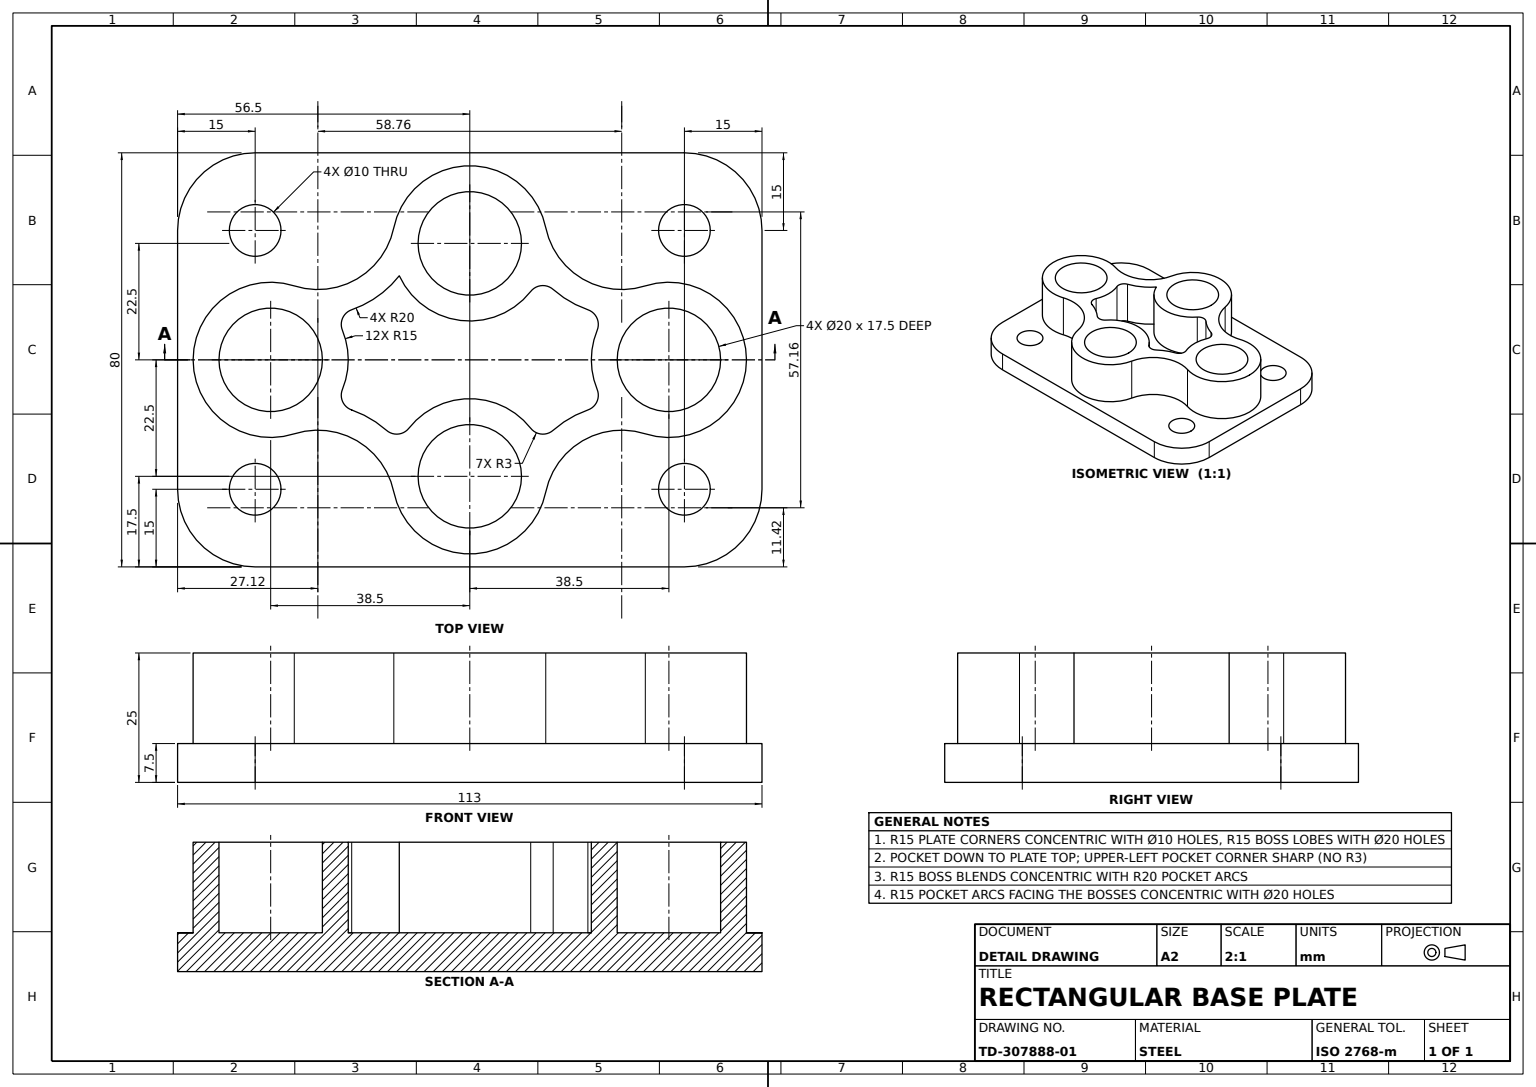
solid
v1 (5.704384,25,-24.627005)
v2 (9.680147,25,-22.833948)
e1 v1 v2 CIRCLE(AX(P(6.845261,25,-21.852406),D(0,-1,0),D(0,0,1)),3)
v3 (5.704384,7.5,-24.627005)
e2 v3 v1 LINE
v4 (9.680147,7.5,-22.833948)
e3 v4 v3 CIRCLE(AX(P(6.845261,7.5,-21.852406),D(0,1,0),D(0,0,1)),3)
e4 v2 v4 LINE
face CYL(AX(P(6.845261,25,-21.852406),D(0,1,0),D(0,0,1)),3) rev [-e1 -e2 -e3 -e4]
v5 (-9.680147,7.5,22.833948)
v6 (-6.845261,7.5,24.852406)
e5 v5 v6 CIRCLE(AX(P(-6.845261,7.5,21.852406),D(0,1,0),D(0,0,1)),3)
v7 (-9.680147,25,22.833948)
e6 v7 v5 LINE
v8 (-6.845261,25,24.852406)
e7 v8 v7 CIRCLE(AX(P(-6.845261,25,21.852406),D(0,-1,0),D(0,0,1)),3)
e8 v6 v8 LINE
face CYL(AX(P(-6.845261,25,21.852406),D(0,1,0),D(0,0,1)),3) rev [-e5 -e6 -e7 -e8]
v9 (0,25,-53.5)
v10 (0,7.5,-53.5)
e9 v9 v10 LINE
v11 (14.289691,25,-33.938781)
e10 v11 v9 CIRCLE(AX(P(0,25,-38.5),D(0,1,0),D(0,0,1)),15)
v12 (14.289691,7.5,-33.938781)
e11 v11 v12 LINE
e12 v12 v10 CIRCLE(AX(P(0,7.5,-38.5),D(0,1,0),D(0,0,1)),15)
face CYL(AX(P(0,25,-38.5),D(0,-1,0),D(0,0,-1)),15) [-e9 -e10 e11 e12]
v13 (25.539691,25,14.688781)
v14 (25.539691,7.5,14.688781)
e13 v13 v14 LINE
v15 (25.539691,7.5,-14.688781)
e14 v14 v15 CIRCLE(AX(P(22.5,7.5,0),D(0,1,0),D(0,0,1)),15)
v16 (25.539691,25,-14.688781)
e15 v16 v15 LINE
e16 v13 v16 CIRCLE(AX(P(22.5,25,0),D(0,1,0),D(0,0,1)),15)
face CYL(AX(P(22.5,25,0),D(0,-1,0),D(0,0,-1)),15) [e13 e14 -e15 -e16]
v17 (0,7.5,28.5)
v18 (0,7.5,48.5)
e17 v17 v18 CIRCLE(AX(P(0,7.5,38.5),D(0,1,0),D(0,0,1)),10)
v19 (0,25,28.5)
e18 v17 v19 LINE
v20 (0,25,48.5)
e19 v19 v20 CIRCLE(AX(P(0,25,38.5),D(0,1,0),D(0,0,1)),10)
e20 v18 v20 LINE
face CYL(AX(P(0,7.5,38.5),D(0,1,0),D(0,0,1)),10) rev [-e17 e18 e19 -e20]
v21 (-40,0,-41.5)
v22 (-25,0,-56.5)
e21 v21 v22 CIRCLE(AX(P(-25,0,-41.5),D(0,-1,0),D(0,0,1)),15)
v23 (-40,7.5,-41.5)
e22 v23 v21 LINE
v24 (-25,7.5,-56.5)
e23 v24 v23 CIRCLE(AX(P(-25,7.5,-41.5),D(0,1,0),D(0,0,1)),15)
e24 v22 v24 LINE
face CYL(AX(P(-25,7.5,-41.5),D(0,-1,0),D(0,0,-1)),15) [-e21 -e22 -e23 -e24]
v25 (25,0,-46.5)
v26 (25,7.5,-46.5)
e25 v25 v26 LINE
v27 (25,7.5,-36.5)
e26 v26 v27 CIRCLE(AX(P(25,7.5,-41.5),D(0,1,0),D(0,0,1)),5)
v28 (25,0,-36.5)
e27 v28 v27 LINE
e28 v25 v28 CIRCLE(AX(P(25,0,-41.5),D(0,1,0),D(0,0,1)),5)
face CYL(AX(P(25,-10,-41.5),D(0,1,0),D(0,0,1)),5) rev [e25 e26 -e27 -e28]
e29 v12 v15 CIRCLE(AX(P(28.579383,7.5,-29.377561),D(0,1,0),D(0,0,1)),15)
e30 v11 v16 CIRCLE(AX(P(28.579383,25,-29.377561),D(0,1,0),D(0,0,1)),15)
face CYL(AX(P(28.579383,25,-29.377561),D(0,-1,0),D(0,0,-1)),15) rev [e15 -e29 -e11 e30]
v29 (14.289691,7.5,33.938781)
e31 v14 v29 CIRCLE(AX(P(28.579383,7.5,29.377561),D(0,1,0),D(0,0,1)),15)
v30 (14.289691,25,33.938781)
e32 v13 v30 CIRCLE(AX(P(28.579383,25,29.377561),D(0,1,0),D(0,0,1)),15)
e33 v30 v29 LINE
face CYL(AX(P(28.579383,25,29.377561),D(0,-1,0),D(0,0,-1)),15) rev [-e31 -e13 e32 e33]
e34 v18 v17 CIRCLE(AX(P(0,7.5,38.5),D(0,1,0),D(0,0,1)),10)
face PLANE(AX(P(0,7.5,38.5),D(0,1,0),D(0,0,1))) [e34 e17]
v31 (-25,0,36.5)
v32 (-25,7.5,36.5)
e35 v31 v32 LINE
v33 (-25,0,46.5)
e36 v33 v31 CIRCLE(AX(P(-25,0,41.5),D(0,1,0),D(0,0,1)),5)
v34 (-25,7.5,46.5)
e37 v33 v34 LINE
e38 v34 v32 CIRCLE(AX(P(-25,7.5,41.5),D(0,1,0),D(0,0,1)),5)
face CYL(AX(P(-25,-10,41.5),D(0,1,0),D(0,0,1)),5) rev [-e35 -e36 e37 e38]
v35 (40,0,41.5)
v36 (25,0,56.5)
e39 v35 v36 CIRCLE(AX(P(25,0,41.5),D(0,-1,0),D(0,0,1)),15)
v37 (40,7.5,41.5)
e40 v37 v35 LINE
v38 (25,7.5,56.5)
e41 v38 v37 CIRCLE(AX(P(25,7.5,41.5),D(0,1,0),D(0,0,1)),15)
e42 v36 v38 LINE
face CYL(AX(P(25,7.5,41.5),D(0,-1,0),D(0,0,-1)),15) [-e39 -e40 -e41 -e42]
v39 (6.845261,7.5,24.852406)
v40 (6.845261,25,24.852406)
e43 v39 v40 LINE
v41 (5.704384,7.5,24.627005)
e44 v41 v39 CIRCLE(AX(P(6.845261,7.5,21.852406),D(0,1,0),D(0,0,1)),3)
v42 (5.704384,25,24.627005)
e45 v42 v41 LINE
e46 v40 v42 CIRCLE(AX(P(6.845261,25,21.852406),D(0,-1,0),D(0,0,1)),3)
face CYL(AX(P(6.845261,25,21.852406),D(0,1,0),D(0,0,1)),3) rev [-e43 -e44 -e45 -e46]
v43 (-25.539691,7.5,-14.688781)
v44 (-25.539691,7.5,14.688781)
e47 v43 v44 CIRCLE(AX(P(-22.5,7.5,0),D(0,1,0),D(0,0,1)),15)
v45 (-14.289691,7.5,-33.938781)
e48 v43 v45 CIRCLE(AX(P(-28.579383,7.5,-29.377561),D(0,1,0),D(0,0,1)),15)
e49 v10 v45 CIRCLE(AX(P(0,7.5,-38.5),D(0,1,0),D(0,0,1)),15)
v46 (-14.289691,7.5,33.938781)
e50 v46 v29 CIRCLE(AX(P(0,7.5,38.5),D(0,1,0),D(0,0,1)),15)
e51 v46 v44 CIRCLE(AX(P(-28.579383,7.5,29.377561),D(0,1,0),D(0,0,1)),15)
v47 (-25,7.5,-46.5)
v48 (-25,7.5,-36.5)
e52 v47 v48 CIRCLE(AX(P(-25,7.5,-41.5),D(0,1,0),D(0,0,1)),5)
e53 v48 v47 CIRCLE(AX(P(-25,7.5,-41.5),D(0,1,0),D(0,0,1)),5)
v49 (25,7.5,36.5)
v50 (25,7.5,46.5)
e54 v49 v50 CIRCLE(AX(P(25,7.5,41.5),D(0,1,0),D(0,0,1)),5)
e55 v50 v49 CIRCLE(AX(P(25,7.5,41.5),D(0,1,0),D(0,0,1)),5)
e56 v32 v34 CIRCLE(AX(P(-25,7.5,41.5),D(0,1,0),D(0,0,1)),5)
e57 v27 v26 CIRCLE(AX(P(25,7.5,-41.5),D(0,1,0),D(0,0,1)),5)
v51 (-40,7.5,41.5)
v52 (-25,7.5,56.5)
e58 v51 v52 CIRCLE(AX(P(-25,7.5,41.5),D(0,1,0),D(0,0,1)),15)
e59 v52 v38 LINE
v53 (40,7.5,-41.5)
e60 v37 v53 LINE
v54 (25,7.5,-56.5)
e61 v53 v54 CIRCLE(AX(P(25,7.5,-41.5),D(0,1,0),D(0,0,1)),15)
e62 v54 v24 LINE
e63 v23 v51 LINE
face PLANE(AX(P(0,7.5,0),D(0,1,0),D(0,0,1))) [-e47 e48 -e49 -e12 e29 -e14 e31 -e50 e51] [-e52 -e53] [-e54 -e55] [-e38 -e56] [-e57 -e26] [e58 e59 e41 e60 e61 e62 e23 e63]
v55 (-25.539691,25,-14.688781)
v56 (-14.289691,25,-33.938781)
e64 v55 v56 CIRCLE(AX(P(-28.579383,25,-29.377561),D(0,1,0),D(0,0,1)),15)
e65 v56 v45 LINE
e66 v55 v43 LINE
face CYL(AX(P(-28.579383,25,-29.377561),D(0,-1,0),D(0,0,-1)),15) rev [e64 e65 -e48 -e66]
v57 (25,0,46.5)
e67 v57 v50 LINE
v58 (25,0,36.5)
e68 v58 v57 CIRCLE(AX(P(25,0,41.5),D(0,1,0),D(0,0,1)),5)
e69 v58 v49 LINE
face CYL(AX(P(25,-10,41.5),D(0,1,0),D(0,0,1)),5) rev [e54 -e67 -e68 e69]
v59 (13.212856,25,-11.779175)
v60 (13.212856,7.5,-11.779175)
e70 v59 v60 LINE
v61 (13.212856,7.5,11.779175)
e71 v60 v61 CIRCLE(AX(P(22.5,7.5,0),D(0,1,0),D(0,0,1)),15)
v62 (13.212856,25,11.779175)
e72 v61 v62 LINE
e73 v59 v62 CIRCLE(AX(P(22.5,25,0),D(0,1,0),D(0,0,1)),15)
face CYL(AX(P(22.5,25,0),D(0,-1,0),D(0,0,-1)),15) [e70 e71 e72 -e73]
v63 (-16.24524,7.5,13.633708)
v64 (-13.212856,7.5,-11.779175)
e74 v63 v64 CIRCLE(AX(P(-22.5,7.5,0),D(0,1,0),D(0,0,1)),15)
e75 v5 v63 CIRCLE(AX(P(-28.579383,7.5,29.377561),D(0,1,0),D(0,0,1)),20)
v65 (-5.704384,7.5,24.627005)
e76 v6 v65 CIRCLE(AX(P(-6.845261,7.5,21.852406),D(0,1,0),D(0,0,1)),3)
v66 (0,7.5,23.5)
e77 v66 v65 CIRCLE(AX(P(0,7.5,38.5),D(0,1,0),D(0,0,1)),15)
e78 v41 v66 CIRCLE(AX(P(0,7.5,38.5),D(0,1,0),D(0,0,1)),15)
v67 (9.680147,7.5,22.833948)
e79 v39 v67 CIRCLE(AX(P(6.845261,7.5,21.852406),D(0,1,0),D(0,0,1)),3)
v68 (13.60203,7.5,16.123169)
e80 v68 v67 CIRCLE(AX(P(28.579383,7.5,29.377561),D(0,1,0),D(0,0,1)),20)
e81 v68 v61 CIRCLE(AX(P(11.355428,7.5,14.13501),D(0,1,0),D(0,0,1)),3)
v69 (13.60203,7.5,-16.123169)
e82 v60 v69 CIRCLE(AX(P(11.355428,7.5,-14.13501),D(0,1,0),D(0,0,1)),3)
e83 v4 v69 CIRCLE(AX(P(28.579383,7.5,-29.377561),D(0,1,0),D(0,0,1)),20)
v70 (-5.704384,7.5,-24.627005)
e84 v70 v3 CIRCLE(AX(P(0,7.5,-38.5),D(0,1,0),D(0,0,1)),15)
v71 (-9.680147,7.5,-22.833948)
e85 v70 v71 CIRCLE(AX(P(-6.845261,7.5,-21.852406),D(0,1,0),D(0,0,1)),3)
v72 (-13.60203,7.5,-16.123169)
e86 v72 v71 CIRCLE(AX(P(-28.579383,7.5,-29.377561),D(0,1,0),D(0,0,1)),20)
e87 v72 v64 CIRCLE(AX(P(-11.355428,7.5,-14.13501),D(0,1,0),D(0,0,1)),3)
face PLANE(AX(P(0,7.5,0),D(0,1,0),D(0,0,1))) [-e74 -e75 e5 e76 -e77 -e78 e44 e79 -e80 e81 -e71 e82 -e83 e3 -e84 e85 -e86 e87]
v73 (-13.212856,25,-11.779175)
e88 v64 v73 LINE
v74 (-13.60203,25,-16.123169)
e89 v74 v72 LINE
e90 v73 v74 CIRCLE(AX(P(-11.355428,25,-14.13501),D(0,-1,0),D(0,0,1)),3)
face CYL(AX(P(-11.355428,25,-14.13501),D(0,1,0),D(0,0,1)),3) rev [-e88 -e87 -e89 -e90]
v75 (0,7.5,-28.5)
v76 (0,7.5,-48.5)
e91 v75 v76 CIRCLE(AX(P(0,7.5,-38.5),D(0,1,0),D(0,0,1)),10)
e92 v76 v75 CIRCLE(AX(P(0,7.5,-38.5),D(0,1,0),D(0,0,1)),10)
face PLANE(AX(P(0,7.5,-38.5),D(0,1,0),D(0,0,1))) [e91 e92]
v77 (0,25,-48.5)
e93 v76 v77 LINE
v78 (0,25,-28.5)
e94 v77 v78 CIRCLE(AX(P(0,25,-38.5),D(0,1,0),D(0,0,1)),10)
e95 v75 v78 LINE
face CYL(AX(P(0,7.5,-38.5),D(0,1,0),D(0,0,1)),10) rev [e93 e94 -e95 -e92]
v79 (-5.704384,25,-24.627005)
e96 v79 v1 CIRCLE(AX(P(0,25,-38.5),D(0,1,0),D(0,0,1)),15)
e97 v79 v70 LINE
face CYL(AX(P(0,25,-38.5),D(0,-1,0),D(0,0,-1)),15) [-e96 e97 e84 e2]
e98 v57 v58 CIRCLE(AX(P(25,0,41.5),D(0,1,0),D(0,0,1)),5)
face CYL(AX(P(25,-10,41.5),D(0,1,0),D(0,0,1)),5) rev [-e98 e67 e55 -e69]
v80 (-5.704384,25,24.627005)
e99 v80 v8 CIRCLE(AX(P(-6.845261,25,21.852406),D(0,-1,0),D(0,0,1)),3)
e100 v65 v80 LINE
face CYL(AX(P(-6.845261,25,21.852406),D(0,1,0),D(0,0,1)),3) rev [e8 -e99 -e100 -e76]
v81 (-16.24524,25,13.633708)
e101 v81 v63 LINE
e102 v7 v81 CIRCLE(AX(P(-28.579383,25,29.377561),D(0,1,0),D(0,0,1)),20)
face CYL(AX(P(-28.579383,25,29.377561),D(0,-1,0),D(0,0,-1)),20) [-e101 -e102 e6 e75]
v82 (-22.5,7.5,-10)
v83 (-22.5,25,-10)
e103 v82 v83 LINE
v84 (-22.5,7.5,10)
e104 v84 v82 CIRCLE(AX(P(-22.5,7.5,0),D(0,1,0),D(0,0,1)),10)
v85 (-22.5,25,10)
e105 v84 v85 LINE
e106 v85 v83 CIRCLE(AX(P(-22.5,25,0),D(0,1,0),D(0,0,1)),10)
face CYL(AX(P(-22.5,7.5,0),D(0,1,0),D(0,0,1)),10) rev [-e103 -e104 e105 e106]
v86 (-14.289691,25,33.938781)
e107 v86 v30 CIRCLE(AX(P(0,25,38.5),D(0,1,0),D(0,0,1)),15)
e108 v86 v46 LINE
face CYL(AX(P(0,25,38.5),D(0,-1,0),D(0,0,-1)),15) [-e107 e108 e50 -e33]
e109 v82 v84 CIRCLE(AX(P(-22.5,7.5,0),D(0,1,0),D(0,0,1)),10)
face PLANE(AX(P(-22.5,7.5,0),D(0,1,0),D(0,0,1))) [e104 e109]
v87 (-25,0,56.5)
e110 v52 v87 LINE
v88 (-40,0,41.5)
e111 v88 v51 LINE
e112 v87 v88 CIRCLE(AX(P(-25,0,41.5),D(0,-1,0),D(0,0,1)),15)
face CYL(AX(P(-25,7.5,41.5),D(0,-1,0),D(0,0,-1)),15) [-e110 -e58 -e111 -e112]
v89 (25,0,-56.5)
e113 v54 v89 LINE
v90 (40,0,-41.5)
e114 v90 v53 LINE
e115 v89 v90 CIRCLE(AX(P(25,0,-41.5),D(0,-1,0),D(0,0,1)),15)
face CYL(AX(P(25,7.5,-41.5),D(0,-1,0),D(0,0,-1)),15) [-e113 -e61 -e114 -e115]
e116 v83 v85 CIRCLE(AX(P(-22.5,25,0),D(0,1,0),D(0,0,1)),10)
face CYL(AX(P(-22.5,7.5,0),D(0,1,0),D(0,0,1)),10) rev [e116 -e105 -e109 e103]
v91 (-9.680147,25,-22.833948)
e117 v71 v91 LINE
e118 v74 v91 CIRCLE(AX(P(-28.579383,25,-29.377561),D(0,1,0),D(0,0,1)),20)
face CYL(AX(P(-28.579383,25,-29.377561),D(0,-1,0),D(0,0,-1)),20) [e89 e86 e117 -e118]
v92 (-25.539691,25,14.688781)
e119 v92 v44 LINE
e120 v55 v92 CIRCLE(AX(P(-22.5,25,0),D(0,1,0),D(0,0,1)),15)
face CYL(AX(P(-22.5,25,0),D(0,-1,0),D(0,0,-1)),15) [e47 -e119 -e120 e66]
e121 v86 v92 CIRCLE(AX(P(-28.579383,25,29.377561),D(0,1,0),D(0,0,1)),15)
face CYL(AX(P(-28.579383,25,29.377561),D(0,-1,0),D(0,0,-1)),15) rev [-e108 e121 e119 -e51]
e122 v31 v33 CIRCLE(AX(P(-25,0,41.5),D(0,1,0),D(0,0,1)),5)
face CYL(AX(P(-25,-10,41.5),D(0,1,0),D(0,0,1)),5) rev [e35 e56 -e37 -e122]
v93 (9.680147,25,22.833948)
e123 v93 v40 CIRCLE(AX(P(6.845261,25,21.852406),D(0,-1,0),D(0,0,1)),3)
e124 v67 v93 LINE
face CYL(AX(P(6.845261,25,21.852406),D(0,1,0),D(0,0,1)),3) rev [-e79 e43 -e123 -e124]
e125 v21 v88 LINE
face PLANE(AX(P(-40,7.5,-56.5),D(1,0,0),D(0,0,-1))) rev [e111 -e63 e22 e125]
v94 (13.60203,25,-16.123169)
e126 v2 v94 CIRCLE(AX(P(28.579383,25,-29.377561),D(0,1,0),D(0,0,1)),20)
e127 v94 v59 CIRCLE(AX(P(11.355428,25,-14.13501),D(0,-1,0),D(0,0,1)),3)
v95 (13.60203,25,16.123169)
e128 v62 v95 CIRCLE(AX(P(11.355428,25,14.13501),D(0,-1,0),D(0,0,1)),3)
e129 v95 v93 CIRCLE(AX(P(28.579383,25,29.377561),D(0,1,0),D(0,0,1)),20)
v96 (0,25,23.5)
e130 v42 v96 CIRCLE(AX(P(0,25,38.5),D(0,1,0),D(0,0,1)),15)
e131 v96 v80 CIRCLE(AX(P(0,25,38.5),D(0,1,0),D(0,0,1)),15)
e132 v81 v73 CIRCLE(AX(P(-22.5,25,0),D(0,1,0),D(0,0,1)),15)
e133 v91 v79 CIRCLE(AX(P(-6.845261,25,-21.852406),D(0,-1,0),D(0,0,1)),3)
e134 v9 v56 CIRCLE(AX(P(0,25,-38.5),D(0,1,0),D(0,0,1)),15)
e135 v20 v19 CIRCLE(AX(P(0,25,38.5),D(0,1,0),D(0,0,1)),10)
v97 (22.5,25,-10)
v98 (22.5,25,10)
e136 v97 v98 CIRCLE(AX(P(22.5,25,0),D(0,1,0),D(0,0,1)),10)
e137 v98 v97 CIRCLE(AX(P(22.5,25,0),D(0,1,0),D(0,0,1)),10)
e138 v78 v77 CIRCLE(AX(P(0,25,-38.5),D(0,1,0),D(0,0,1)),10)
face PLANE(AX(P(0,25,0),D(0,1,0),D(0,0,1))) [e96 e1 e126 e127 e73 e128 e129 e123 e46 e130 e131 e99 e7 e102 e132 e90 e118 e133] [-e106 -e116] [-e121 e107 -e32 e16 -e30 e10 e134 -e64 e120] [-e19 -e135] [-e136 -e137] [-e138 -e94]
v99 (22.5,7.5,-10)
v100 (22.5,7.5,10)
e139 v99 v100 CIRCLE(AX(P(22.5,7.5,0),D(0,1,0),D(0,0,1)),10)
e140 v100 v99 CIRCLE(AX(P(22.5,7.5,0),D(0,1,0),D(0,0,1)),10)
face PLANE(AX(P(22.5,7.5,0),D(0,1,0),D(0,0,1))) [e139 e140]
e141 v95 v68 LINE
face CYL(AX(P(11.355428,25,14.13501),D(0,1,0),D(0,0,1)),3) rev [-e72 -e81 -e141 -e128]
face CYL(AX(P(-22.5,25,0),D(0,-1,0),D(0,0,-1)),15) [e74 e88 -e132 e101]
e142 v69 v94 LINE
face CYL(AX(P(11.355428,25,-14.13501),D(0,1,0),D(0,0,1)),3) rev [-e70 -e127 -e142 -e82]
face CYL(AX(P(28.579383,25,-29.377561),D(0,-1,0),D(0,0,-1)),20) [-e126 e4 e83 e142]
v101 (-25,0,-36.5)
e143 v101 v48 LINE
v102 (-25,0,-46.5)
e144 v102 v47 LINE
e145 v101 v102 CIRCLE(AX(P(-25,0,-41.5),D(0,1,0),D(0,0,1)),5)
face CYL(AX(P(-25,-10,-41.5),D(0,1,0),D(0,0,1)),5) rev [e143 e53 -e144 -e145]
e146 v87 v36 LINE
face PLANE(AX(P(-40,7.5,56.5),D(0,0,-1),D(-1,0,0))) rev [e110 e146 e42 -e59]
e147 v102 v101 CIRCLE(AX(P(-25,0,-41.5),D(0,1,0),D(0,0,1)),5)
face CYL(AX(P(-25,-10,-41.5),D(0,1,0),D(0,0,1)),5) rev [e52 -e143 -e147 e144]
face CYL(AX(P(-6.845261,25,-21.852406),D(0,1,0),D(0,0,1)),3) rev [-e85 -e97 -e133 -e117]
e148 v99 v97 LINE
e149 v100 v98 LINE
face CYL(AX(P(22.5,7.5,0),D(0,1,0),D(0,0,1)),10) rev [-e139 e148 e136 -e149]
e150 v96 v66 LINE
face CYL(AX(P(0,25,38.5),D(0,-1,0),D(0,0,-1)),15) [e100 -e131 e150 e77]
face CYL(AX(P(28.579383,25,29.377561),D(0,-1,0),D(0,0,-1)),20) [e124 -e129 e141 e80]
e151 v28 v25 CIRCLE(AX(P(25,0,-41.5),D(0,1,0),D(0,0,1)),5)
e152 v89 v22 LINE
e153 v35 v90 LINE
face PLANE(AX(P(0,0,0),D(0,1,0),D(0,0,1))) rev [e98 e68] [e122 e36] [e28 e151] [e147 e145] [-e125 e21 -e152 e115 -e153 e39 -e146 e112]
face CYL(AX(P(25,-10,-41.5),D(0,1,0),D(0,0,1)),5) rev [e57 -e25 -e151 e27]
face CYL(AX(P(0,25,-38.5),D(0,-1,0),D(0,0,-1)),15) [e9 e49 -e65 -e134]
face CYL(AX(P(22.5,7.5,0),D(0,1,0),D(0,0,1)),10) rev [-e148 -e140 e149 e137]
face CYL(AX(P(0,25,38.5),D(0,-1,0),D(0,0,-1)),15) [e45 e78 -e150 -e130]
face PLANE(AX(P(40,7.5,0),D(-1,0,0),D(0,0,1))) rev [e114 -e60 e40 e153]
face PLANE(AX(P(40,7.5,-56.5),D(0,0,1),D(1,0,0))) rev [e113 e152 e24 -e62]
face CYL(AX(P(0,7.5,38.5),D(0,1,0),D(0,0,1)),10) rev [e20 e135 -e18 -e34]
face CYL(AX(P(0,7.5,-38.5),D(0,1,0),D(0,0,1)),10) rev [e95 e138 -e93 -e91]
